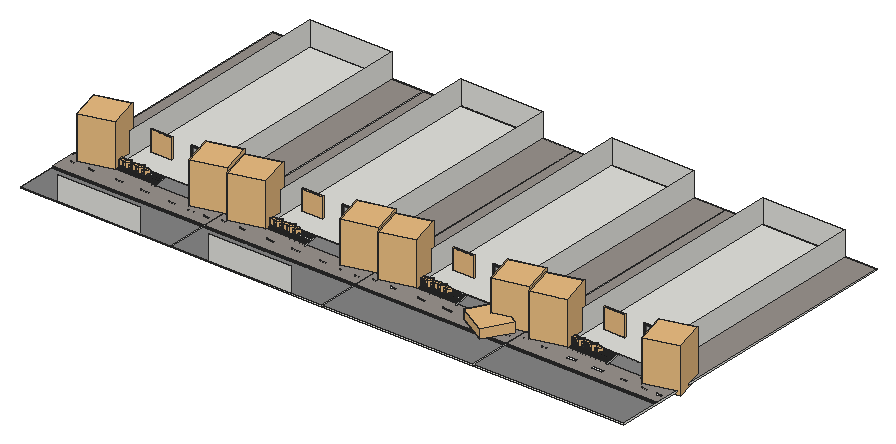
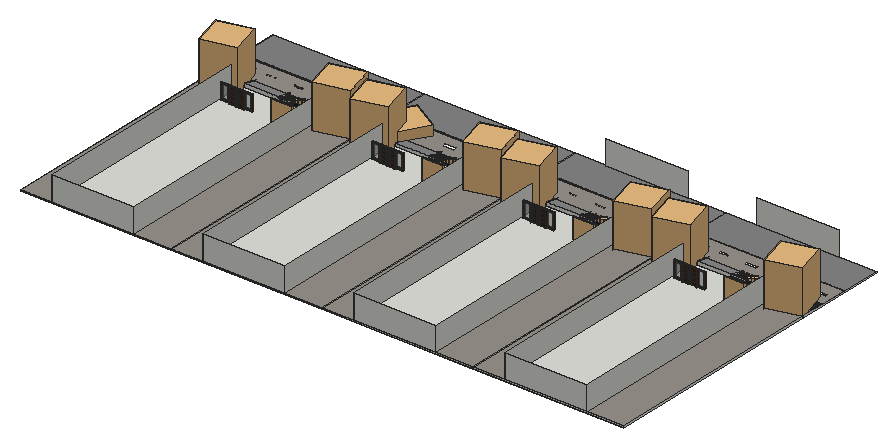
# SketchUp Ruby script. Lengths in inches.
U = 1.inch
M = Sketchup.active_model
def pt(a) = Geom::Point3d.new(a.map { |v| v * U })
def face(e, loops, mat)
  f = e.add_face(loops[0].map { |a| pt(a) })
  loops[1..].each { |l| e.add_face(l.map { |a| pt(a) }).erase! }
  f.material = f.back_material = mat if mat
  f
end
# faces: each face lists its corners as indices into pts; further lists are holes
def faces(e, pts, list, mat = nil) = list.each { |f| face(e, (f[0].is_a?(Array) ? f : [f]).map { |l| l.map { |i| pts[i] } }, mat) }
# xy, xz, yz: faces in a plane at the given z, y or x. An outline is a flat list of corners, or four numbers for a rectangle; further outlines are holes
def ring(l) = l.size == 4 ? [[l[0], l[1]], [l[2], l[1]], [l[2], l[3]], [l[0], l[3]]] : l.each_slice(2).to_a
def flat(e, list, mat, &to3) = list.each { |f| face(e, (f[0].is_a?(Array) ? f : [f]).map { |l| ring(l).map { |u, v| to3.(u, v) } }, mat) }
def xy(e, z, list, mat = nil) = flat(e, list, mat) { |x, y| [x, y, z] }
def xz(e, y, list, mat = nil) = flat(e, list, mat) { |x, z| [x, y, z] }
def yz(e, x, list, mat = nil) = flat(e, list, mat) { |y, z| [x, y, z] }
def lines(e, pts, list) = list.each { |a, b| e.add_line(pt(pts[a]), pt(pts[b])) }
# prism: a flat outline (further loops are holes) pulled along v
def prism(e, loops, v, mat = nil)
  f = face(e, loops, mat); d = Geom::Vector3d.new(v.map { |x| x * U })
  f.pushpull(f.normal.samedirection?(d) ? d.length : -d.length)
end
def box(e, o, s, mat = nil) = prism(e, [[o, [o[0] + s[0], o[1], o[2]], [o[0] + s[0], o[1] + s[1], o[2]], [o[0], o[1] + s[1], o[2]]]], [0, 0, s[2]], mat)
def at(x, y, z, deg = 0) = Geom::Transformation.translation(pt([x, y, z])) * Geom::Transformation.rotation(ORIGIN, Z_AXIS, deg.degrees)
def axes(o, x, y, z) = Geom::Transformation.new([*x, 0, *y, 0, *z, 0, *pt(o).to_a, 1])
def part(name) = M.definitions.add(name)
# library, detail: a bought-in or finely detailed component or shape, given as its bounding box
def library(name, o, s) = part(name).tap { |d| box(d.entities, o, s) }
def detail(e, o, s) = box(e.add_group.entities, o, s)
def put(e, d, t, mat = nil) = e.add_instance(d, t).tap { |i| i.material = mat if mat }
def group(e, t, mat = nil) = e.add_group.tap { |g| g.transformation = t; g.material = mat if mat }.entities
root = M.entities
M.materials.add("Color_000").color = [255, 255, 255]
M.materials.add("MADEIRAS PORTAS MOD 4").color = [48, 37, 30]
M.materials.add("Material__1").color = [95, 70, 46]
M.materials.add("[Aluminum]").color = [179, 179, 179]
M.materials.add("[Color M07]").color = [58, 58, 58]
M.materials.add("[Color M08]").color = [30, 30, 30]
M.materials.add("[Granite Dark Gray]").color = [38, 37, 37]
M.materials.add("[Granite Tile]").color = [153, 146, 141]
M.materials.add("[Tile Grey]").color = [132, 132, 132]
M.materials.add("[Tile Grey]1").color = [133, 133, 133]
M.materials.add("[Translucent Glass Gray]").color = [128, 128, 128]
M.materials["[Translucent Glass Gray]"].alpha = 0.5
M.materials.add("[Wood Veneer 01]").color = [66, 38, 20]
c1 = library("002+Bmw+M4+++mat3.4+2017",[-252.8,19.48,9.01],[196.94,171.32,55.15])
c2 = part("Untitled (5)")
xy(c2.entities,0,[[[158.81,26.5625,306.06,993.3125],[226.57,518.17,239.57,583.92],[225.28,357.51,237.28,411.51],[222.61,182.28,236.36,226.53],[239.71,931.55,251.46,972.3],[233.64,703.93,242.14,755.18],[240.05,835.03,248.8,880.53],[222.04,66.5,231.29,100.5]]])
xy(c2.entities,0,[[222.04,66.5,231.29,100.5],[222.61,182.28,236.36,226.53],[225.28,357.51,237.28,411.51],[226.57,518.17,239.57,583.92],[233.64,703.93,242.14,755.18],
  [240.05,835.03,248.8,880.53],[239.71,931.55,251.46,972.3]],"Color_000")
c3 = library("Areca palm plant",[0,0,0],[49.1,36.6,54.46])
c4 = library("Group\#74",[-84.69,-90.07,-0.36],[176.51,175.13,171.4])
c5 = library("Group38\#2",[14.01,28.44,-23.43],[18.58,18.32,38.89])
c6 = library("Group\#130",[-7.34,-1.2,0],[38.67,35.81,49.04])
c7 = library("Group20\#1",[-20.81,-17.08,3.79],[39.86,39.43,37.51])
c8 = part("Group\#3")
xy(c8.entities,0,[[0,0,6,234.8],[30,0,36,234.8]])
xy(c8.entities,3,[[6,0,30,234.8]])
xy(c8.entities,7,[[6,5,30,229.8]],"Material__1")
xy(c8.entities,15,[[[0,0,36,234.8],[6,5,30,229.8]]])
xz(c8.entities,0,[[0,0,6,0,6,3,30,3,30,0,36,0,36,15,0,15]])
xz(c8.entities,5,[[6,7,30,15]])
xz(c8.entities,229.8,[[6,7,30,15]])
xz(c8.entities,234.8,[[0,0,0,15,36,15,36,0,30,0,30,3,6,3,6,0]])
yz(c8.entities,0,[[0,0,234.8,15]])
yz(c8.entities,6,[[0,0,234.8,3],[5,7,229.8,15]])
yz(c8.entities,30,[[0,0,234.8,3],[5,7,229.8,15]])
yz(c8.entities,36,[[0,0,234.8,15]])
c9 = part("Planted trough")
put(c9.entities,c3,axes([-6.2,158.41,6.08],[0.45017,-0.56191,0],[0.66137,0.52986,0],[0,0,0.72]))
put(c9.entities,c3,axes([-6.2,56.6,6.08],[0.45017,-0.56191,0],[0.66137,0.52986,0],[0,0,0.72]))
put(c9.entities,c4,axes([17.19,15.79,6.07],[-0.08133,-0.14087,0],[0.14087,-0.08133,0],[0,0,0.1725]))
put(c9.entities,c4,axes([14.93,173.12,6.05],[-0.04961,-0.08593,0],[0.08593,-0.04961,0],[0,0,0.10522]))
put(c9.entities,c4,axes([17.19,223.04,6.07],[-0.08133,-0.14087,0],[0.14087,-0.08133,0],[0,0,0.1725]))
put(c9.entities,c5,axes([-4.1,-1.15,28.17],[0.8848,0,0],[0,0.94674,0],[0,0,0.85826]))
put(c9.entities,c4,axes([14.93,193.18,6.05],[-0.04961,-0.08593,0],[0.08593,-0.04961,0],[0,0,0.10522]))
put(c9.entities,c4,axes([14.93,91.37,6.05],[-0.04961,-0.08593,0],[0.08593,-0.04961,0],[0,0,0.10522]))
put(c9.entities,c6,axes([24.9375,191.72,8],[0,0.79,0],[-0.79,0,0],[0,0,0.79]))
put(c9.entities,c7,axes([18.97,181.79,4.77],[0,0.85,0],[-0.85,0,0],[0,0,0.85]))
put(c9.entities,c4,axes([14.93,145.87,6.05],[-0.04961,-0.08593,0],[0.08593,-0.04961,0],[0,0,0.10522]))
put(c9.entities,c7,axes([18.97,79.98,4.77],[0,0.85,0],[-0.85,0,0],[0,0,0.85]))
put(c9.entities,c4,axes([14.93,71.3,6.05],[-0.04961,-0.08593,0],[0.08593,-0.04961,0],[0,0,0.10522]))
put(c9.entities,c6,axes([24.9375,89.91,8],[0,0.79,0],[-0.79,0,0],[0,0,0.79]))
put(c9.entities,c4,axes([14.93,44.05,6.05],[-0.04961,-0.08593,0],[0.08593,-0.04961,0],[0,0,0.10522]))
put(c9.entities,c4,axes([17.19,121.23,6.07],[-0.08133,-0.14087,0],[0.14087,-0.08133,0],[0,0,0.1725]))
put(c9.entities,c8,at(0,0,0),"[Color M07]")
put(c9.entities,c5,axes([-4.1,100.66,28.17],[0.8848,0,0],[0,0.94674,0],[0,0,0.85826]))
c10 = library("Palm tree",[-4.09,-4.52,0],[193.52,193.51,258.93])
c11 = part("Palm+Tree")
put(c11.entities,c10,at(25.51,-21.81,0,15))
c12 = library("Curtains",[0,0,0],[121.73,8.19,117.22])
c13 = part("Component\#9")
prism(c13.entities,[[[23.23,0,0],[0,0,0],[0,0,74.02],[23.23,0,74.02]],[[2.76,0,2.76],[20.47,0,2.76],[20.47,0,71.26],[3.07,0,71.26]]],[0,1.38,0],"[Wood Veneer 01]")
c14 = part("Component\#1")
g1 = group(c14.entities,at(20.87,-0.79,28.35))
xy(g1,0,[[0,0,1.18,0.79]],"[Aluminum]")
xy(g1,23.62,[[0,0,1.18,0.79]],"[Aluminum]")
xz(g1,0,[[0,0,1.18,23.62]],"MADEIRAS PORTAS MOD 4")
xz(g1,0.79,[[0,0,1.18,23.62]],"[Aluminum]")
yz(g1,0,[[0,0,0.79,23.62]],"[Aluminum]")
yz(g1,1.18,[[0,0,0.79,23.62]],"[Aluminum]")
g2 = group(c14.entities,at(0,0,0),"MADEIRAS PORTAS MOD 4")
xy(g2,0,[[0,0,23.62,1.57]],"[Wood Veneer 01]")
xy(g2,80.31,[[0,0,23.62,1.57]],"[Wood Veneer 01]")
xz(g2,0,[[0,0,17.32,19.78],[17.32,0,17.32,19.78,0,19.78,0,20.18,17.32,20.18,17.32,39.96,0,39.96,0,40.35,17.32,40.35,17.32,60.14,0,60.14,0,60.53,17.32,60.53,17.32,80.31,17.72,80.31,17.72,0],[17.72,0,23.62,80.31],[0,20.18,17.32,39.96],[0,40.35,17.32,60.14],
  [0,60.53,17.32,80.31]],"[Wood Veneer 01]")
xz(g2,1.57,[[0,0,17.32,19.78],[17.32,0,17.72,0,17.72,80.31,17.32,80.31,17.32,60.53,0,60.53,0,60.14,17.32,60.14,17.32,40.35,0,40.35,0,39.96,17.32,39.96,17.32,20.18,0,20.18,0,19.78,17.32,19.78],[17.72,0,23.62,80.31],[0,20.18,17.32,39.96],[0,40.35,17.32,60.14],
  [0,60.53,17.32,80.31]],"[Wood Veneer 01]")
yz(g2,0,[[0,0,1.57,80.31]],"[Wood Veneer 01]")
yz(g2,23.62,[[0,0,1.57,80.31]],"[Wood Veneer 01]")
g3 = group(c14.entities,at(20.87,2.36,28.35))
box(g3,[0,-0.79,0],[1.18,0.79,23.62],"[Aluminum]")
c15 = part("Component\#8")
xz(c15.entities,2.95,[[-20.47,9.06,-2.76,77.56],[54.72,9.06,72.44,77.56]],"[Translucent Glass Gray]")
put(c15.entities,c13,at(-23.23,2.26,6.3),"MADEIRAS PORTAS MOD 4")
put(c15.entities,c13,axes([75.2,2.26,6.3],[-1,0,0],[0,1,0],[0,0,1]))
put(c15.entities,c14,at(2.36,2.17,0),"MADEIRAS PORTAS MOD 4")
put(c15.entities,c14,axes([49.61,2.17,0],[-1,0,0],[0,1,0],[0,0,1]))
g4 = group(c15.entities,at(0,0,0),"MADEIRAS PORTAS MOD 4")
xy(g4,0,[[0,0,2.36,5.91],[49.61,0,51.97,5.91]],"[Wood Veneer 01]")
xy(g4,3.9375,[[-25.59,0,0,5.91],[51.97,0,77.56,5.91]],"[Wood Veneer 01]")
xy(g4,6.3,[[-23.23,0,0,5.91],[51.97,0,75.2,5.91]],"[Wood Veneer 01]")
xy(g4,80.31,[[-23.23,0,0,5.91],[2.36,0,49.61,5.91],[51.97,0,75.2,5.91]],"[Wood Veneer 01]")
xy(g4,82.68,[[-25.59,0,77.56,5.91]],"[Wood Veneer 01]")
xz(g4,0,[[[0,0,2.36,0,2.36,80.31,49.61,80.31,49.61,0,51.97,0,51.97,3.9375,77.56,3.9375,77.56,82.68,-25.59,82.68,-25.59,3.9375,0,3.9375,0,6.3,-23.23,6.3,-23.23,80.31,0,80.31],[51.97,6.3,75.2,80.31]]],"MADEIRAS PORTAS MOD 4")
xz(g4,5.91,[[[0,0,2.36,0,2.36,80.31,49.61,80.31,49.61,0,51.97,0,51.97,3.9375,77.56,3.9375,77.56,82.68,-25.59,82.68,-25.59,3.9375,0,3.9375,0,6.3,-23.23,6.3,-23.23,80.31,0,80.31],[51.97,6.3,75.2,80.31]]],"[Wood Veneer 01]")
yz(g4,-25.59,[[0,3.9375,5.91,82.68]],"[Wood Veneer 01]")
yz(g4,-23.23,[[0,6.3,5.91,80.31]],"[Wood Veneer 01]")
yz(g4,0,[[0,0,5.91,3.9375],[0,3.9375,5.91,6.3],[0,6.3,5.91,80.31]],"[Wood Veneer 01]")
yz(g4,2.36,[[0,0,5.91,80.31]],"[Wood Veneer 01]")
yz(g4,49.61,[[0,0,5.91,80.31]],"[Wood Veneer 01]")
yz(g4,51.97,[[0,0,5.91,3.9375],[0,3.9375,5.91,6.3],[0,6.3,5.91,80.31]],"[Wood Veneer 01]")
yz(g4,75.2,[[0,6.3,5.91,80.31]],"[Wood Veneer 01]")
yz(g4,77.56,[[0,3.9375,5.91,82.68]],"[Wood Veneer 01]")
c16 = part("Wood+Door (2)")
put(c16.entities,c15,at(25.59,0,0),"MADEIRAS PORTAS MOD 4")
xy(root,-18.8125,[[1.85,1835.625,880.6,3671.25],[880.6,1835.625,1759.35,3671.25],[1759.35,1835.625,2638.1,3671.25],[2638.1,1835.625,3516.85,3671.25]])
xy(root,-13.3125,[[395.95,2263.9375,463.7,2274],[1274.7,2263.9375,1342.45,2274],[2153.45,2263.9375,2221.2,2274],[3032.2,2263.9375,3099.95,2274],[395.95,2274,463.7,2285.625],
  [1274.7,2274,1342.45,2285.625],[2153.45,2274,2221.2,2285.625],[3032.2,2274,3099.95,2285.625]])
xy(root,-11.3125,[[480.15,2205.875,678.9,2205.875,678.9,2294.125,493.86,2294.125,493.86,2218.17,480.15,2218.17],[1358.9,2205.875,1557.65,2205.875,1557.65,2294.125,1372.61,2294.125,1372.61,2218.17,1358.9,2218.17],[2237.65,2205.875,2436.4,2205.875,2436.4,2294.125,2251.36,2294.125,2251.36,2218.17,2237.65,2218.17],[3116.4,2205.875,3315.15,2205.875,3315.15,2294.125,3130.11,2294.125,3130.11,2218.17,3116.4,2218.17],[479.03,2218.17,480.15,2263.9375],
  [480.15,2218.17,493.86,2294.125],[1357.78,2218.17,1358.9,2263.9375],[1358.9,2218.17,1372.61,2294.125],[2236.53,2218.17,2237.65,2263.9375],[2237.65,2218.17,2251.36,2294.125],
  [3115.28,2218.17,3116.4,2263.9375],[3116.4,2218.17,3130.11,2294.125],[463.7,2263.9375,479.03,2274],[479.03,2263.9375,480.15,2274],[1342.45,2263.9375,1357.78,2274],
  [1357.78,2263.9375,1358.9,2274],[2221.2,2263.9375,2236.53,2274],[2236.53,2263.9375,2237.65,2274],[3099.95,2263.9375,3115.28,2274],[3115.28,2263.9375,3116.4,2274],
  [463.7,2274,479.03,2285.625],[479.03,2274,480.15,2285.625],[1342.45,2274,1357.78,2285.625],[1357.78,2274,1358.9,2285.625],[2221.2,2274,2236.53,2285.625],
  [2236.53,2274,2237.65,2285.625],[3099.95,2274,3115.28,2285.625],[3115.28,2274,3116.4,2285.625],[479.03,2285.625,480.15,2285.625,480.15,2294.125,698.16,2294.125,698.16,3671.25,218.97,3671.25,218.97,2294.125,479.03,2294.125],[1357.78,2285.625,1358.9,2285.625,1358.9,2294.125,1576.91,2294.125,1576.91,3671.25,1097.72,3671.25,1097.72,2294.125,1357.78,2294.125],
  [2236.53,2285.625,2237.65,2285.625,2237.65,2294.125,2455.66,2294.125,2455.66,3671.25,1976.47,3671.25,1976.47,2294.125,2236.53,2294.125],[3115.28,2285.625,3116.4,2285.625,3116.4,2294.125,3334.41,2294.125,3334.41,3671.25,2855.22,3671.25,2855.22,2294.125,3115.28,2294.125]])
xy(root,-11.3125,[[1.85,2062.38,880.6,2062.38,880.6,2294.125,678.9,2294.125,678.9,2205.875,480.15,2205.875,480.15,2218.17,1.85,2218.17],[880.6,2062.38,1759.35,2062.38,1759.35,2294.125,1557.65,2294.125,1557.65,2205.875,1358.9,2205.875,1358.9,2218.17,880.6,2218.17],[1759.35,2062.38,2638.1,2062.38,2638.1,2294.125,2436.4,2294.125,2436.4,2205.875,2237.65,2205.875,2237.65,2218.17,1759.35,2218.17],[2638.1,2062.38,3516.85,2062.38,3516.85,2294.125,3315.15,2294.125,3315.15,2205.875,3116.4,2205.875,3116.4,2218.17,2638.1,2218.17]],"[Granite Dark Gray]")
xy(root,-11.3125,[[1.85,2294.125,218.97,3671.25],[698.16,2294.125,880.6,3671.25],[880.6,2294.125,1097.72,3671.25],[1576.91,2294.125,1759.35,3671.25],[1759.35,2294.125,1976.47,3671.25],
  [2455.66,2294.125,2638.1,3671.25],[2638.1,2294.125,2855.22,3671.25],[3334.41,2294.125,3516.85,3671.25]],"[Granite Tile]")
xy(root,-11.3125,[[1.85,1835.625,880.6,2062.38],[880.6,1835.625,1759.35,2062.38],[1759.35,1835.625,2638.1,2062.38],[2638.1,1835.625,3516.85,2062.38]],"[Tile Grey]1")
xy(root,-9.1875,[[1.85,2218.17,479.03,2294.125],[880.6,2218.17,1357.78,2294.125],[1759.35,2218.17,2236.53,2294.125],[2638.1,2218.17,3115.28,2294.125]],"[Granite Dark Gray]")
xy(root,-7.25,[[395.95,2274,480.15,2285.625],[1274.7,2274,1358.9,2285.625],[2153.45,2274,2237.65,2285.625],[3032.2,2274,3116.4,2285.625],[395.95,2285.625,480.15,2294.125],
  [1274.7,2285.625,1358.9,2294.125],[2153.45,2285.625,2237.65,2294.125],[3032.2,2285.625,3116.4,2294.125]])
xy(root,-3.25,[[395.95,2263.9375,480.15,2274],[1274.7,2263.9375,1358.9,2274],[2153.45,2263.9375,2237.65,2274],[3032.2,2263.9375,3116.4,2274]])
xy(root,0,[[395.95,2285.625,480.15,2294.125],[1274.7,2285.625,1358.9,2294.125],[2153.45,2285.625,2237.65,2294.125],[3032.2,2285.625,3116.4,2294.125]])
xy(root,3.25,[[395.95,2274,480.15,2285.625],[1274.7,2274,1358.9,2285.625],[2153.45,2274,2237.65,2285.625],[3032.2,2274,3116.4,2285.625]])
xz(root,1835.625,[[218.97,-11.3125,698.16,128.5],[1097.72,-11.3125,1576.91,128.5]])
xz(root,2218.17,[[1.85,-11.3125,379.41,-9.1875],[379.41,-11.3125,479.03,-9.1875],[479.03,-11.3125,493.86,-11.3125,479.03,-9.1875],[880.6,-11.3125,1258.16,-9.1875],[1258.16,-11.3125,1357.78,-9.1875],
  [1357.78,-11.3125,1372.61,-11.3125,1357.78,-9.1875],[1759.35,-11.3125,2136.91,-9.1875],[2136.91,-11.3125,2236.53,-9.1875],[2236.53,-11.3125,2251.36,-11.3125,2236.53,-9.1875],[2638.1,-11.3125,3015.66,-9.1875],
  [3015.66,-11.3125,3115.28,-9.1875],[3115.28,-11.3125,3130.11,-11.3125,3115.28,-9.1875]])
xz(root,2263.9375,[[395.95,-13.3125,463.7,-13.3125,463.7,-11.3125,480.15,-11.3125,480.15,-3.25,395.95,-3.25],[1274.7,-13.3125,1342.45,-13.3125,1342.45,-11.3125,1358.9,-11.3125,1358.9,-3.25,1274.7,-3.25],[2153.45,-13.3125,2221.2,-13.3125,2221.2,-11.3125,2237.65,-11.3125,2237.65,-3.25,2153.45,-3.25],[3032.2,-13.3125,3099.95,-13.3125,3099.95,-11.3125,3116.4,-11.3125,3116.4,-3.25,3032.2,-3.25]],"[Color M08]")
xz(root,2274,[[395.95,-7.25,480.15,-3.25],[1274.7,-7.25,1358.9,-3.25],[2153.45,-7.25,2237.65,-3.25],[3032.2,-7.25,3116.4,-3.25]])
xz(root,2274,[[395.95,-3.25,480.15,3.25],[1274.7,-3.25,1358.9,3.25],[2153.45,-3.25,2237.65,3.25],[3032.2,-3.25,3116.4,3.25]],"[Color M08]")
xz(root,2285.625,[[395.95,-13.3125,395.95,-7.25,480.15,-7.25,480.15,-11.3125,463.7,-11.3125,463.7,-13.3125],[1274.7,-13.3125,1274.7,-7.25,1358.9,-7.25,1358.9,-11.3125,1342.45,-11.3125,1342.45,-13.3125],[2153.45,-13.3125,2153.45,-7.25,2237.65,-7.25,2237.65,-11.3125,2221.2,-11.3125,2221.2,-13.3125],[3032.2,-13.3125,3032.2,-7.25,3116.4,-7.25,3116.4,-11.3125,3099.95,-11.3125,3099.95,-13.3125],[395.95,0,480.15,3.25],
  [1274.7,0,1358.9,3.25],[2153.45,0,2237.65,3.25],[3032.2,0,3116.4,3.25]])
xz(root,2285.625,[[395.95,3.25,480.15,8.5],[1274.7,3.25,1358.9,8.5],[2153.45,3.25,2237.65,8.5],[3032.2,3.25,3116.4,8.5]],"[Color M08]")
xz(root,2294.125,[[1.85,-11.3125,218.97,-9.1875],[218.97,-11.3125,395.95,-9.1875],[395.95,-11.3125,463.7,-9.1875],[463.7,-11.3125,479.03,-9.1875],[480.15,-11.3125,480.15,-9.35,493.86,-11.3125],
  [493.86,-11.3125,678.9,-11.3125,678.9,8.5,480.15,8.5,480.15,-9.35],[880.6,-11.3125,1097.72,-9.1875],[1097.72,-11.3125,1274.7,-9.1875],[1274.7,-11.3125,1342.45,-9.1875],[1342.45,-11.3125,1357.78,-9.1875],
  [1358.9,-11.3125,1358.9,-9.35,1372.61,-11.3125],[1372.61,-11.3125,1557.65,-11.3125,1557.65,8.5,1358.9,8.5,1358.9,-9.35],[1759.35,-11.3125,1976.47,-9.1875],[1976.47,-11.3125,2153.45,-9.1875],[2153.45,-11.3125,2221.2,-9.1875],
  [2221.2,-11.3125,2236.53,-9.1875],[2237.65,-11.3125,2237.65,-9.35,2251.36,-11.3125],[2251.36,-11.3125,2436.4,-11.3125,2436.4,8.5,2237.65,8.5,2237.65,-9.35],[2638.1,-11.3125,2855.22,-9.1875],[2855.22,-11.3125,3032.2,-9.1875],
  [3032.2,-11.3125,3099.95,-9.1875],[3099.95,-11.3125,3115.28,-9.1875],[3116.4,-11.3125,3116.4,-9.35,3130.11,-11.3125],[3130.11,-11.3125,3315.15,-11.3125,3315.15,8.5,3116.4,8.5,3116.4,-9.35],[395.95,-9.1875,463.7,-7.25],
  [1274.7,-9.1875,1342.45,-7.25],[2153.45,-9.1875,2221.2,-7.25],[3032.2,-9.1875,3099.95,-7.25],[395.95,-7.25,480.15,0],[1274.7,-7.25,1358.9,0],
  [2153.45,-7.25,2237.65,0],[3032.2,-7.25,3116.4,0],[395.95,0,480.15,8.5],[1274.7,0,1358.9,8.5],[2153.45,0,2237.65,8.5],
  [3032.2,0,3116.4,8.5]])
xz(root,2294.125,[[480.15,-9.35,480.15,-7.25,463.7,-7.25,463.7,-9.1875,479.03,-9.1875],[1358.9,-9.35,1358.9,-7.25,1342.45,-7.25,1342.45,-9.1875,1357.78,-9.1875],[2237.65,-9.35,2237.65,-7.25,2221.2,-7.25,2221.2,-9.1875,2236.53,-9.1875],[3116.4,-9.35,3116.4,-7.25,3099.95,-7.25,3099.95,-9.1875,3115.28,-9.1875]],"[Color M07]")
xz(root,2294.125,[[218.97,-9.1875,395.95,8.5],[1097.72,-9.1875,1274.7,8.5],[1976.47,-9.1875,2153.45,8.5],[2855.22,-9.1875,3032.2,8.5]],"[Color M08]")
xz(root,2294.125,[[678.9,-11.3125,698.16,118.38],[1557.65,-11.3125,1576.91,118.38],[2436.4,-11.3125,2455.66,118.38],[3315.15,-11.3125,3334.41,118.38]],"[Wood Veneer 01]")
xz(root,3671.25,[[1.85,-18.8125,880.6,-11.3125],[880.6,-18.8125,1759.35,-11.3125],[1759.35,-18.8125,2638.1,-11.3125],[2638.1,-18.8125,3516.85,-11.3125],[218.97,-11.3125,698.16,128.5],
  [1097.72,-11.3125,1576.91,128.5],[1976.47,-11.3125,2455.66,128.5],[2855.22,-11.3125,3334.41,128.5]])
yz(root,1.85,[[1835.625,-18.8125,1835.625,-11.3125,2218.17,-11.3125,2218.17,-9.1875,2294.125,-9.1875,2294.125,-11.3125,3671.25,-11.3125,3671.25,-18.8125]])
yz(root,218.97,[[2294.125,-11.3125,2294.125,8.5,2358.81,8.5,2358.81,128.5,3671.25,128.5,3671.25,-11.3125]])
yz(root,395.95,[[2263.9375,-13.3125,2274,-11.3125],[2274,-13.3125,2285.625,-11.3125],[2263.9375,-11.3125,2274,-3.25],[2274,-11.3125,2285.625,-7.25],[2274,-7.25,2285.625,3.25],
  [2285.625,-7.25,2294.125,0],[2285.625,0,2294.125,8.5]])
yz(root,463.7,[[2263.9375,-13.3125,2274,-11.3125],[2274,-13.3125,2285.625,-11.3125]])
yz(root,479.03,[[2218.17,-11.3125,2294.125,-9.1875]])
yz(root,480.15,[[2205.875,-11.3125,2285.625,6.59,2285.625,3.25,2274,3.25,2274,-3.25,2263.9375,-3.25,2263.9375,-11.3125],[2263.9375,-11.3125,2285.625,-11.3125,2285.625,-7.25,2274,-7.25,2274,-3.25,2263.9375,-3.25],[2285.625,-11.3125,2294.125,-7.25],[2285.625,0,2285.625,6.59,2294.125,8.5,2294.125,0],[2285.625,6.59,2294.125,8.5,2285.625,8.5]])
yz(root,678.9,[[2205.875,-11.3125,2294.125,-11.3125,2294.125,8.5]])
yz(root,698.16,[[2294.125,-11.3125,3671.25,128.5]])
yz(root,880.6,[[1835.625,-18.8125,3671.25,-11.3125],[2218.17,-11.3125,2294.125,-9.1875]])
yz(root,1097.72,[[2294.125,-11.3125,2294.125,8.5,2358.81,8.5,2358.81,128.5,3671.25,128.5,3671.25,-11.3125]])
yz(root,1274.7,[[2263.9375,-13.3125,2274,-11.3125],[2274,-13.3125,2285.625,-11.3125],[2263.9375,-11.3125,2274,-3.25],[2274,-11.3125,2285.625,-7.25],[2274,-7.25,2285.625,3.25],
  [2285.625,-7.25,2294.125,0],[2285.625,0,2294.125,8.5]])
yz(root,1342.45,[[2263.9375,-13.3125,2274,-11.3125],[2274,-13.3125,2285.625,-11.3125]])
yz(root,1357.78,[[2218.17,-11.3125,2294.125,-9.1875]])
yz(root,1358.9,[[2205.875,-11.3125,2285.625,6.59,2285.625,3.25,2274,3.25,2274,-3.25,2263.9375,-3.25,2263.9375,-11.3125],[2263.9375,-11.3125,2285.625,-11.3125,2285.625,-7.25,2274,-7.25,2274,-3.25,2263.9375,-3.25],[2285.625,-11.3125,2294.125,-7.25],[2285.625,0,2285.625,6.59,2294.125,8.5,2294.125,0],[2285.625,6.59,2294.125,8.5,2285.625,8.5]])
yz(root,1557.65,[[2205.875,-11.3125,2294.125,-11.3125,2294.125,8.5]])
yz(root,1576.91,[[2294.125,-11.3125,3671.25,128.5]])
yz(root,1759.35,[[1835.625,-18.8125,3671.25,-11.3125],[2218.17,-11.3125,2294.125,-9.1875]])
yz(root,1976.47,[[2294.125,-11.3125,2294.125,8.5,2358.81,8.5,2358.81,128.5,3671.25,128.5,3671.25,-11.3125]])
yz(root,2153.45,[[2263.9375,-13.3125,2274,-11.3125],[2274,-13.3125,2285.625,-11.3125],[2263.9375,-11.3125,2274,-3.25],[2274,-11.3125,2285.625,-7.25],[2274,-7.25,2285.625,3.25],
  [2285.625,-7.25,2294.125,0],[2285.625,0,2294.125,8.5]])
yz(root,2221.2,[[2263.9375,-13.3125,2274,-11.3125],[2274,-13.3125,2285.625,-11.3125]])
yz(root,2236.53,[[2218.17,-11.3125,2294.125,-9.1875]])
yz(root,2237.65,[[2205.875,-11.3125,2285.625,6.59,2285.625,3.25,2274,3.25,2274,-3.25,2263.9375,-3.25,2263.9375,-11.3125],[2263.9375,-11.3125,2285.625,-11.3125,2285.625,-7.25,2274,-7.25,2274,-3.25,2263.9375,-3.25],[2285.625,-11.3125,2294.125,-7.25],[2285.625,0,2285.625,6.59,2294.125,8.5,2294.125,0],[2285.625,6.59,2294.125,8.5,2285.625,8.5]])
yz(root,2436.4,[[2205.875,-11.3125,2294.125,-11.3125,2294.125,8.5]])
yz(root,2455.66,[[2294.125,-11.3125,3671.25,128.5]])
yz(root,2638.1,[[1835.625,-18.8125,3671.25,-11.3125],[2218.17,-11.3125,2294.125,-9.1875]])
yz(root,2855.22,[[2294.125,-11.3125,2294.125,8.5,2358.81,8.5,2358.81,128.5,3671.25,128.5,3671.25,-11.3125]])
yz(root,3032.2,[[2263.9375,-13.3125,2274,-11.3125],[2274,-13.3125,2285.625,-11.3125],[2263.9375,-11.3125,2274,-3.25],[2274,-11.3125,2285.625,-7.25],[2274,-7.25,2285.625,3.25],
  [2285.625,-7.25,2294.125,0],[2285.625,0,2294.125,8.5]])
yz(root,3099.95,[[2263.9375,-13.3125,2274,-11.3125],[2274,-13.3125,2285.625,-11.3125]])
yz(root,3115.28,[[2218.17,-11.3125,2294.125,-9.1875]])
yz(root,3116.4,[[2205.875,-11.3125,2285.625,6.59,2285.625,3.25,2274,3.25,2274,-3.25,2263.9375,-3.25,2263.9375,-11.3125],[2263.9375,-11.3125,2285.625,-11.3125,2285.625,-7.25,2274,-7.25,2274,-3.25,2263.9375,-3.25],[2285.625,-11.3125,2294.125,-7.25],[2285.625,0,2285.625,6.59,2294.125,8.5,2294.125,0],[2285.625,6.59,2294.125,8.5,2285.625,8.5]])
yz(root,3315.15,[[2205.875,-11.3125,2294.125,-11.3125,2294.125,8.5]])
yz(root,3334.41,[[2294.125,-11.3125,3671.25,128.5]])
yz(root,3516.85,[[1835.625,-18.8125,3671.25,-11.3125]])
p = [[678.9,2205.875,-11.3125],[678.9,2294.125,8.5],[481.29,2294.125,8.5],[480.15,2294.125,8.5],[480.15,2285.625,6.59],[480.15,2205.875,-11.3125],
  [1557.65,2205.875,-11.3125],[1557.65,2294.125,8.5],[1360.04,2294.125,8.5],[1358.9,2294.125,8.5],[1358.9,2285.625,6.59],[1358.9,2205.875,-11.3125],
  [2436.4,2205.875,-11.3125],[2436.4,2294.125,8.5],[2238.79,2294.125,8.5],[2237.65,2294.125,8.5],[2237.65,2285.625,6.59],[2237.65,2205.875,-11.3125],
  [3315.15,2205.875,-11.3125],[3315.15,2294.125,8.5],[3117.54,2294.125,8.5],[3116.4,2294.125,8.5],[3116.4,2285.625,6.59],[3116.4,2205.875,-11.3125],
  [480.15,2294.125,-9.35],[479.03,2294.125,-9.1875],[479.03,2218.17,-9.1875],[493.86,2218.17,-11.3125],[493.86,2294.125,-11.3125],[1358.9,2294.125,-9.35],
  [1357.78,2294.125,-9.1875],[1357.78,2218.17,-9.1875],[1372.61,2218.17,-11.3125],[1372.61,2294.125,-11.3125],[2237.65,2294.125,-9.35],[2236.53,2294.125,-9.1875],
  [2236.53,2218.17,-9.1875],[2251.36,2218.17,-11.3125],[2251.36,2294.125,-11.3125],[3116.4,2294.125,-9.35],[3115.28,2294.125,-9.1875],[3115.28,2218.17,-9.1875],
  [3130.11,2218.17,-11.3125],[3130.11,2294.125,-11.3125],[2221.2,2294.125,-11.3125],[2221.2,2285.625,-11.3125],[2153.45,2294.125,-11.3125],[2153.45,2285.625,-11.3125],
  [3032.2,2294.125,-11.3125],[3032.2,2285.625,-11.3125],[3099.95,2294.125,-11.3125],[3099.95,2285.625,-11.3125],[463.7,2294.125,-11.3125],[463.7,2285.625,-11.3125],
  [395.95,2294.125,-11.3125],[395.95,2285.625,-11.3125],[1274.7,2294.125,-11.3125],[1274.7,2285.625,-11.3125],[1342.45,2294.125,-11.3125],[1342.45,2285.625,-11.3125]]
faces(root,p,[[0,1,2,3,4,5],[6,7,8,9,10,11],[12,13,14,15,16,17],[18,19,20,21,22,23]],"[Tile Grey]")
faces(root,p,[[24,25,26,27,28],[29,30,31,32,33],[34,35,36,37,38],[39,40,41,42,43]])
lines(root,p,[[44,45],[46,47],[48,49],[50,51],[52,53],[54,55],[56,57],[58,59]])
put(root,c1,at(2565.55,1978.9,-11.3125,-30))
put(root,c2,axes([1733.3,2382.9,-7.22],[0,-1,0],[0.91088,0,0],[0,0,1]),"[Granite Tile]")
put(root,c2,axes([854.55,2382.9,-7.22],[0,-1,0],[0.91088,0,0],[0,0,1]),"[Granite Tile]")
put(root,c2,axes([-24.2,2382.9,-7.22],[0,-1,0],[0.91088,0,0],[0,0,1]),"[Granite Tile]")
put(root,c2,axes([2612.05,2382.9,-7.22],[0,-1,0],[0.91088,0,0],[0,0,1]),"[Granite Tile]")
put(root,c9,axes([1275.73,2262.37,-7.25],[0,0.7469,0],[-0.7469,0,0],[0,0,0.7469]))
put(root,c9,axes([3033.23,2262.37,-7.25],[0,0.7469,0],[-0.7469,0,0],[0,0,0.7469]))
put(root,c9,axes([2154.48,2262.37,-7.25],[0,0.7469,0],[-0.7469,0,0],[0,0,0.7469]))
put(root,c9,axes([396.98,2262.37,-7.25],[0,0.7469,0],[-0.7469,0,0],[0,0,0.7469]))
put(root,c11,at(1569.52,2201.3,-29.65))
put(root,c11,at(3327.02,2201.3,-29.65))
put(root,c11,at(2448.27,2201.3,-29.65))
put(root,c11,at(690.77,2201.3,-29.65))
put(root,c11,at(2668,2204.7,-20.67))
put(root,c11,at(1789.25,2204.7,-20.67))
put(root,c11,at(910.5,2204.7,-20.67))
put(root,c11,at(31.75,2204.7,-20.67))
put(root,c12,at(2022.96,2458.74,-9.86))
put(root,c12,at(1144.21,2458.74,-9.86))
put(root,c12,at(265.46,2458.74,-9.86))
put(root,c12,at(2901.71,2458.74,-9.86))
put(root,c16,axes([2246.4,2468.68,0],[1.75378,0,0],[0,1,0],[0,0,1.16459]))
put(root,c16,axes([488.9,2468.68,0],[1.75378,0,0],[0,1,0],[0,0,1.16459]))
put(root,c16,axes([1367.65,2468.68,0],[1.75378,0,0],[0,1,0],[0,0,1.16459]))
put(root,c16,axes([3125.15,2468.68,0],[1.75378,0,0],[0,1,0],[0,0,1.16459]))
